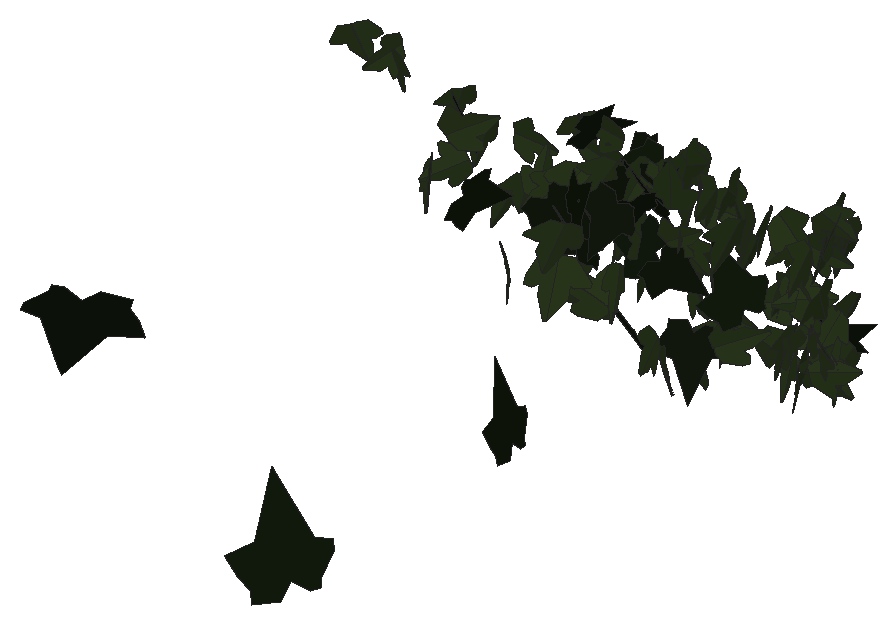
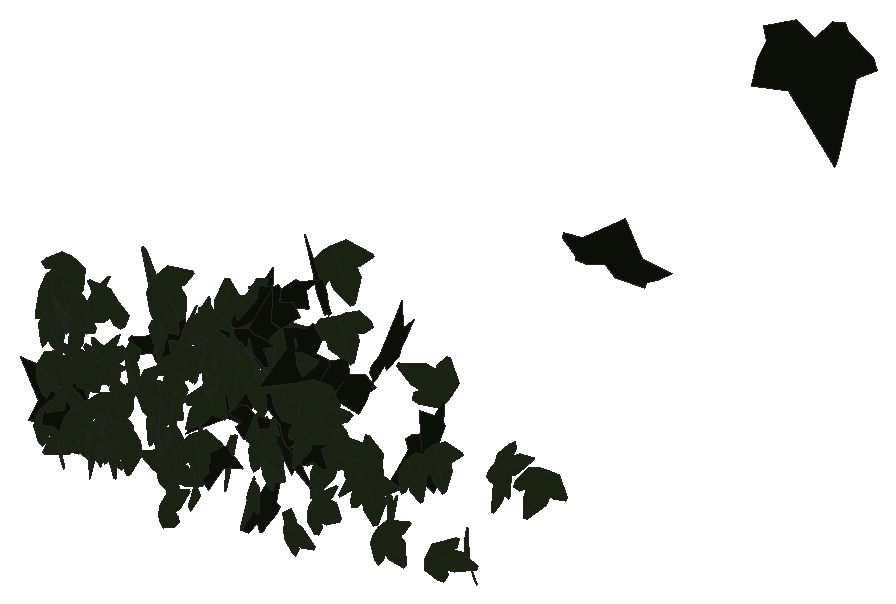
# SketchUp Ruby script. Lengths in inches.
U = 1.inch
M = Sketchup.active_model
def pt(a) = Geom::Point3d.new(a.map { |v| v * U })
def face(e, loops, mat)
  f = e.add_face(loops[0].map { |a| pt(a) })
  loops[1..].each { |l| e.add_face(l.map { |a| pt(a) }).erase! }
  f.material = f.back_material = mat if mat
  f
end
# faces: each face lists its corners as indices into pts; further lists are holes
def faces(e, pts, list, mat = nil) = list.each { |f| face(e, (f[0].is_a?(Array) ? f : [f]).map { |l| l.map { |i| pts[i] } }, mat) }
# xy, xz, yz: faces in a plane at the given z, y or x. An outline is a flat list of corners, or four numbers for a rectangle; further outlines are holes
def ring(l) = l.size == 4 ? [[l[0], l[1]], [l[2], l[1]], [l[2], l[3]], [l[0], l[3]]] : l.each_slice(2).to_a
def flat(e, list, mat, &to3) = list.each { |f| face(e, (f[0].is_a?(Array) ? f : [f]).map { |l| ring(l).map { |u, v| to3.(u, v) } }, mat) }
def xy(e, z, list, mat = nil) = flat(e, list, mat) { |x, y| [x, y, z] }
def xz(e, y, list, mat = nil) = flat(e, list, mat) { |x, z| [x, y, z] }
def yz(e, x, list, mat = nil) = flat(e, list, mat) { |y, z| [x, y, z] }
def lines(e, pts, list) = list.each { |a, b| e.add_line(pt(pts[a]), pt(pts[b])) }
# prism: a flat outline (further loops are holes) pulled along v
def prism(e, loops, v, mat = nil)
  f = face(e, loops, mat); d = Geom::Vector3d.new(v.map { |x| x * U })
  f.pushpull(f.normal.samedirection?(d) ? d.length : -d.length)
end
def box(e, o, s, mat = nil) = prism(e, [[o, [o[0] + s[0], o[1], o[2]], [o[0] + s[0], o[1] + s[1], o[2]], [o[0], o[1] + s[1], o[2]]]], [0, 0, s[2]], mat)
def at(x, y, z, deg = 0) = Geom::Transformation.translation(pt([x, y, z])) * Geom::Transformation.rotation(ORIGIN, Z_AXIS, deg.degrees)
def axes(o, x, y, z) = Geom::Transformation.new([*x, 0, *y, 0, *z, 0, *pt(o).to_a, 1])
def part(name) = M.definitions.add(name)
# library, detail: a bought-in or finely detailed component or shape, given as its bounding box
def library(name, o, s) = part(name).tap { |d| box(d.entities, o, s) }
def detail(e, o, s) = box(e.add_group.entities, o, s)
def put(e, d, t, mat = nil) = e.add_instance(d, t).tap { |i| i.material = mat if mat }
def group(e, t, mat = nil) = e.add_group.tap { |g| g.transformation = t; g.material = mat if mat }.entities
root = M.entities
M.materials.add("efeu1").color = [18, 25, 13]
M.materials.add("efeu2").color = [43, 57, 29]
c1 = part("ivyleaf_9")
p = [[1.54,2.16,1.25],[1.36,2.04,1.19],[-0.21,0.99,0.68],[-0.71,1.11,0.82],[-0.85,0.86,0.67],[-0.8,0.17,0.21],
  [-0.9,-0.01,0.1],[-0.67,-0.16,-0.02],[-0.08,-0.08,-0.05],[-0.03,-0.6,-0.4],[0.65,-0.88,-0.66],[0.83,-0.6,-0.49],
  [1.29,-0.42,-0.43],[1.8125,-0.07,-0.26],[1.21,0.44,0.15]]
faces(c1.entities,p,[[0,1,2,3,4,5,6,7,8,9,10,11,12,13,14]],"efeu1")
c2 = part("ivyleaf_10")
p = [[0,0.5,-0.03],[-0.0625,2.02,-0.43],[-0.19,2.01,-0.46],[-0.54,1.05,-0.29],[-0.52,0.625,-0.18],[-0.83,0.76,-0.28],
  [-1.16,0.64,-0.33],[-1.15,0.33,-0.24],[-0.77,-0.39,0.02],[-0.3,-0.51,0.16],[0.04,-0.48,0.23],[-0.02,2.01,-0.4375],
  [-0.06,2.01,-0.43],[0.04,-0.49,0.23],[0.67,-0.49,0.14],[1.38,0.36,-0.2],[1.375,0.51,-0.24],[0.81,0.65,-0.19],
  [0.62,0.59,-0.15],[0.6,1.09,-0.28],[0.5,1.23,-0.31]]
faces(c2.entities,p,[[0,1,2,3,4,5,6,7,8,9,10],[11,12,0,13,14,15,16,17,18,19,20]],"efeu2")
put(root,c1,axes([502.76,113.14,166.2],[0.63244,0.88262,-0.81674],[-0.4951,-0.63807,-1.10132],[-1.17596,0.74332,0.02443]))
put(root,c1,axes([509.15,115.98,157.04],[-1.26753,-0.11528,0.14381],[0.14961,0.00424,1.22642],[-0.12419,1.18175,0.00963]))
put(root,c1,axes([509.9,126.54,157.74],[-0.12905,-0.74325,0.56709],[0.24711,0.50872,0.7733],[-0.96441,0.22981,0.12226]))
put(root,c2,axes([509.01,130.26,163.54],[-0.45484,-0.62688,0.27611],[-0.14286,-0.23089,-0.78521],[0.72124,-0.44107,0.0186]))
put(root,c2,axes([508.29,130.92,161.64],[0.6186,0.59597,-0.17145],[-0.12286,-0.11932,-0.85966],[-0.65642,0.58397,-0.00068]))
put(root,c1,axes([508,132.13,163.08],[-0.11361,0.32654,0.68893],[0.21953,-0.63048,0.35679],[0.76682,0.22888,-0.00007]))
put(root,c2,axes([509.58,132.42,161.15],[0.62014,-0.35844,0.2759],[0.23589,-0.15102,-0.70387],[0.41988,0.61423,-0.01205]))
put(root,c1,axes([509.11,132.97,163.34],[-0.33636,-0.60165,0.16807],[-0.08252,-0.14242,-0.70457],[0.66773,-0.32067,-0.00242]))
put(root,c2,axes([508.61,132.79,159.72],[0.32026,0.29936,0.67732],[-0.5943,-0.35655,0.43102],[0.49605,-0.62045,0.07911]))
put(root,c2,axes([510.35,133.33,158.47],[0.55725,-0.41938,-0.236],[-0.17229,0.16327,-0.69103],[0.48531,0.53951,0.02567]))
put(root,c1,axes([509.21,133.71,163.17],[0.13784,0.62288,-0.22727],[-0.05689,-0.21225,-0.66119],[-0.71063,0.13781,0.00884]))
put(root,c2,axes([510.51,133.74,157.55],[-0.47497,0.45089,0.29765],[-0.21835,0.20259,-0.65504],[-0.53385,-0.48402,0.0031]))
put(root,c1,axes([505.63,133.89,161.93],[-0.0439,-0.14962,-0.77155],[0.31276,0.68333,-0.15983],[0.75516,-0.29172,0.02134]))
put(root,c2,axes([512.77,134.55,163.07],[-0.10334,-0.73527,0.34378],[-0.04182,-0.34127,-0.74248],[0.81059,-0.11135,0.00552]))
put(root,c2,axes([509.08,134.52,164.03],[0.17112,0.44347,-0.44791],[-0.19418,-0.39233,-0.48893],[-0.63878,0.23806,0.02864]))
put(root,c2,axes([501.59,134.09,162.96],[-0.31468,-0.25699,0.66664],[0.50868,0.43092,0.40624],[-0.50169,0.59812,-0.00625]))
put(root,c1,axes([508.51,133.94,163.68],[0.03435,0.0646,-0.7024],[0.13751,0.66355,0.07224],[0.71973,-0.12986,0.01972]))
put(root,c2,axes([506.11,134.21,159.22],[-0.30045,-0.6959,-0.35345],[0.17015,0.31122,-0.7574],[0.76174,-0.344,0.02977]))
put(root,c1,axes([513.23,134.43,160.41],[-0.71941,-0.3952,0.04042],[0.05266,-0.012,0.82003],[-0.39375,0.72044,0.03582]))
put(root,c2,axes([513.62,134.3,163.61],[0.3742,-0.58447,-0.45342],[-0.24442,0.3819,-0.694],[0.69818,0.44695,0.00006]))
put(root,c1,axes([508.85,134.89,162.64],[0.67994,-0.40982,0.23307],[-0.20003,0.11962,0.79389],[-0.42692,-0.70875,-0.00077]))
put(root,c2,axes([512.63,134.27,158.8125],[-0.1722,-0.2198,0.69867],[0.42346,0.55573,0.27921],[-0.59761,0.45712,-0.00348]))
put(root,c2,axes([502.91,135.06,157.77],[-0.24543,0.14957,0.73666],[0.60331,-0.42307,0.2869],[0.4484,0.6511,0.0172]))
put(root,c1,axes([506.42,135.04,160.11],[0.1436,-0.69547,0.0659],[0.00129,0.06473,0.73626],[-0.75422,-0.13231,0.01381]))
put(root,c2,axes([507.27,135.05,163.17],[-0.34879,-0.56177,0.39572],[-0.20967,-0.33561,-0.66124],[0.65438,-0.40696,-0.00094]))
put(root,c1,axes([501.87,134.21,160.62],[-0.02601,0.15388,-0.76833],[-0.2657,0.72148,0.15349],[0.73717,0.26548,0.02821]))
put(root,c2,axes([509.69,135.1,162.81],[-0.69884,-0.42344,-0.02594],[-0.01628,-0.02319,0.81704],[-0.42392,0.69894,0.01139]))
put(root,c1,axes([510.56,135.21,158.05],[-0.50863,-0.46562,-0.37996],[0.28315,0.25339,-0.68956],[0.53009,-0.58212,0.00376]))
put(root,c2,axes([514.76,135.74,162.17],[-0.06277,-0.3232,0.67328],[0.34516,-0.61172,-0.26147],[0.66229,0.28818,0.20008]))
put(root,c1,axes([509.4375,135.03,160.43],[0.03261,-0.16919,-0.68484],[0.05456,0.65788,-0.17339],[0.73224,-0.04148,0.04341]))
put(root,c1,axes([507.77,135.82,156.68],[0.53818,-0.55853,0.0638],[-0.04252,0.04763,0.77562],[-0.56056,-0.53985,0.00242]))
put(root,c1,axes([500.41,135.98,162.21],[0.20601,-0.41465,0.62014],[0.23799,-0.57321,-0.46233],[0.70702,0.31377,-0.02507]))
put(root,c2,axes([515.69,135.34,161.25],[-0.00186,-0.64236,-0.35691],[-0.00636,0.35691,-0.64233],[0.73482,0.00146,-0.00646]))
put(root,c2,axes([509.45,135.51,161.05],[-0.35965,-0.1338,0.50197],[0.48203,0.18375,0.37323],[-0.24547,0.55686,-0.00254]))
put(root,c2,axes([510.64,135.65,156.45],[-0.43062,0.45422,0.11722],[0.07325,-0.09043,0.62851],[0.5001,0.40436,0.00887]))
put(root,c1,axes([508.54,136.04,163.38],[-0.69456,-0.30587,-0.09091],[0.08487,0.03286,-0.75892],[0.3076,-0.69971,0.0041]))
put(root,c2,axes([514.28,136.11,157.07],[0.08219,-0.45535,-0.49981],[0.14455,-0.48002,0.46109],[-0.6605,-0.16171,0.03871]))
put(root,c2,axes([510.46,136.25,162.76],[-0.09771,-0.0466,0.72839],[0.38966,-0.62473,0.0123],[0.61716,0.38705,0.10756]))
put(root,c1,axes([508.31,135.9,160.12],[-0.49256,-0.24603,-0.52245],[-0.44637,-0.27346,0.54961],[-0.36639,0.66392,0.03277]))
put(root,c2,axes([507.32,136.14,162.03],[-0.24988,-0.35753,0.52872],[-0.28449,-0.44589,-0.43597],[0.57135,-0.37838,0.01416]))
put(root,c2,axes([515.21,136.01,161.87],[0.15719,-0.64001,-0.20308],[0.06404,-0.19332,0.65885],[-0.66839,-0.16904,0.01537]))
put(root,c2,axes([507.68,136.17,160.2],[-0.24466,0.54231,0.45521],[0.18978,-0.41377,0.59493],[0.68213,0.30963,-0.00226]))
put(root,c1,axes([505.57,135.73,159.64],[-0.67893,-0.21061,0.3147],[0.30789,0.06907,0.71047],[-0.22045,0.74513,0.02309]))
put(root,c2,axes([514.97,136.1875,158.62],[-0.19972,-0.04855,0.73188],[0.6946,-0.25623,0.17255],[0.23567,0.71406,0.11168]))
put(root,c2,axes([509.44,136.36,161.77],[0.18407,-0.39832,0.53365],[0.31637,-0.43488,-0.43372],[0.58596,0.35992,0.06654]))
put(root,c2,axes([504.91,136.14,161.58],[0.55503,0.32084,-0.42443],[-0.38423,-0.18256,-0.64045],[-0.36803,0.67444,0.02855]))
put(root,c2,axes([508.58,135.55,162.85],[-0.08432,-0.20978,-0.66626],[0.22283,0.60653,-0.23271],[0.6931,-0.22052,-0.00624]))
put(root,c2,axes([508.26,135.76,162.48],[0.00385,0.00014,0.69704],[-0.65732,0.23193,0.00359],[-0.23192,-0.65733,0.00141]))
put(root,c2,axes([506.5,136.27,160.11],[-0.39587,-0.53806,-0.08489],[-0.03261,-0.08135,0.66764],[-0.54374,0.39661,0.02177]))
put(root,c2,axes([509.75,135.95,160.56],[-0.36927,-0.35019,-0.33316],[0.2699,0.20281,-0.50798],[0.43576,-0.42237,0.03231]))
put(root,c2,axes([514.43,136.54,160.15],[-0.03483,0.05289,0.64535],[-0.27547,-0.5861,0.03317],[0.586,-0.27237,0.05395]))
put(root,c2,axes([513.5625,136.46,158.56],[0.20561,-0.66087,0.29802],[0.10354,-0.27983,-0.69196],[0.71752,0.22975,0.01445]))
put(root,c2,axes([514.16,136.17,160.26],[0.20562,-0.11436,-0.72012],[0.72137,-0.07706,0.21822],[-0.10619,-0.74493,0.08798]))
put(root,c2,axes([515.6,136.26,159.97],[0.59977,-0.08531,-0.20905],[-0.20735,0.02668,-0.60581],[0.08935,0.6346,-0.00263]))
put(root,c2,axes([513.57,136.17,162.82],[0.46659,0.11586,0.59129],[0.57429,0.14078,-0.48076],[-0.18232,0.73994,-0.00112]))
put(root,c2,axes([504.04,136.3125,160.77],[0.51328,0.03697,-0.5499],[-0.54968,-0.0203,-0.51444],[-0.04007,0.75195,0.01315]))
put(root,c2,axes([513.59,136.38,157.62],[0.56688,-0.32942,0.126],[0.10541,-0.06937,-0.65561],[0.33657,0.57656,-0.00689]))
put(root,c2,axes([513.72,136.29,160.6],[0.29138,0.00595,0.60829],[0.60673,0.0458,-0.29108],[-0.04387,0.67292,0.01443]))
put(root,c2,axes([513.69,136.23,158.44],[-0.19042,-0.63364,-0.10714],[0.04502,0.09831,-0.66148],[0.64106,-0.19512,0.01463]))
put(root,c2,axes([515.59,135.93,162.73],[0.22256,-0.29941,0.51724],[-0.26569,0.44483,0.37182],[-0.53534,-0.34524,0.0305]))
put(root,c1,axes([507.7,136.25,163.02],[-0.68079,0.40892,0.16753],[-0.15229,0.07174,-0.79399],[-0.41484,-0.69742,0.01655]))
put(root,c2,axes([511.14,136.37,157.64],[-0.02455,-0.00322,0.68376],[-0.6544,-0.19826,-0.02443],[0.19825,-0.65485,0.00403]))
put(root,c2,axes([509.47,136.54,158.8],[0.11131,-0.06283,0.68473],[0.65079,-0.2143,-0.12546],[0.22198,0.65978,0.02446]))
put(root,c2,axes([511.58,136.43,159.35],[0.13411,-0.72065,0.02541],[0.00289,-0.02531,-0.73302],[0.72109,0.13412,-0.00179]))
put(root,c2,axes([514.98,136.27,157.79],[0.12019,-0.0061,-0.71282],[0.71223,0.03094,0.11983],[0.0295,-0.72222,0.01115]))
put(root,c2,axes([512.75,136.36,158.04],[-0.33329,0.06564,-0.65922],[0.65408,-0.08457,-0.33911],[-0.10519,-0.73383,-0.01989]))
put(root,c1,axes([505.5,135.79,163.63],[0.35688,0.4478,0.5238],[0.33325,0.40416,-0.57258],[-0.60319,0.48824,-0.00643]))
put(root,c2,axes([511.2,136.7,162.79],[-0.22234,0.17606,-0.62368],[0.391,-0.48939,-0.27754],[-0.51681,-0.446,0.05834]))
put(root,c2,axes([514.78,136.39,162.17],[0.01057,-0.04651,0.69636],[0.67818,0.16514,0.00074],[-0.16481,0.67658,0.04769]))
put(root,c2,axes([515.31,136.28,163.66],[-0.44934,-0.1857,-0.41301],[0.37651,0.17006,-0.48609],[0.2516,-0.58614,-0.01018]))
put(root,c2,axes([509.75,136.01,163.8],[0.08521,-0.31214,-0.62246],[0.0305,0.62817,-0.31084],[0.69567,0.0107,0.08987]))
put(root,c2,axes([506.2,136.5,163.4],[-0.16344,0.09841,-0.64148],[-0.64335,0.06241,0.17349],[0.08533,0.65902,0.07936]))
put(root,c2,axes([511.32,136.15,163.31],[0.03194,-0.47522,-0.52635],[-0.01219,0.52644,-0.47603],[0.70903,0.03046,0.01553]))
put(root,c2,axes([514.81,136.35,157.88],[-0.55346,-0.08744,-0.51833],[0.51138,0.08463,-0.56031],[0.12166,-0.75353,-0.00279]))
put(root,c2,axes([506.04,136.38,157.22],[0.00212,0.06646,0.66374],[-0.66611,0.03558,-0.00144],[-0.03555,-0.66279,0.06648]))
put(root,c2,axes([510.59,136.86,157.19],[0.06859,-0.15343,0.55243],[0.36363,-0.41337,-0.16605],[0.47364,0.33958,0.04748]))
put(root,c1,axes([505.58,136.66,161.64],[0.33775,-0.11441,-0.67583],[0.67314,0.19748,0.30298],[0.12929,-0.72926,0.18807]))
put(root,c2,axes([508.91,136.37,162.45],[-0.38907,0.28249,-0.46068],[-0.40035,0.24393,0.47532],[0.40208,0.51623,0.0275]))
put(root,c2,axes([512.88,136.98,159.75],[0.00838,-0.05996,0.64957],[0.3723,-0.53299,-0.05401],[0.53566,0.37139,0.02737]))
put(root,c2,axes([506.82,136.77,160.23],[-0.13343,-0.6181,0.25042],[-0.02977,-0.24961,-0.63195],[0.66623,-0.13495,0.02191]))
put(root,c1,axes([506.07,136.69,160.61],[-0.6226,0.34576,-0.33148],[0.28567,-0.16831,-0.71212],[-0.38448,-0.68496,0.00766]))
put(root,c2,axes([496.7,137.02,163.05],[0.06487,0.12347,-0.66154],[-0.25581,-0.6102,-0.13897],[-0.62245,0.26364,-0.01184]))
put(root,c2,axes([509.23,136.375,163.65],[-0.28923,-0.57839,-0.34318],[0.17542,0.29575,-0.64631],[0.64926,-0.33757,0.02175]))
put(root,c2,axes([498.15,136.93,159.18],[0.38476,-0.31679,0.534],[0.423,-0.32614,-0.49826],[0.45452,0.57169,0.01166]))
put(root,c2,axes([500.66,136.79,161.51],[-0.06195,-0.61475,0.18438],[0.01894,-0.18691,-0.61681],[0.64152,-0.05385,0.03601]))
put(root,c2,axes([505.86,136.77,162.09],[-0.38912,-0.02553,-0.61373],[-0.60901,-0.07879,0.3894],[-0.08017,0.72241,0.02078]))
put(root,c2,axes([515.01,136.15,159.35],[-0.09835,-0.24476,-0.67812],[0.23379,0.63659,-0.26367],[0.68198,-0.25352,-0.00741]))
put(root,c2,axes([515.08,136.66,159.14],[0.59464,-0.21924,-0.29688],[-0.27622,0.10899,-0.63374],[0.24476,0.65563,0.00608]))
put(root,c2,axes([506.36,137.08,159.875],[0.20806,-0.47597,0.46003],[0.17433,-0.4258,-0.5194],[0.63858,0.27132,-0.00809]))
put(root,c2,axes([510.11,137,159.05],[-0.02815,0.0607,-0.71661],[0.51489,-0.499,-0.06249],[-0.5021,-0.5151,-0.0239]))
put(root,c2,axes([514.99,137.05,157.32],[-0.08279,0.07986,0.75173],[0.64319,-0.38991,0.11226],[0.39722,0.64801,-0.0251]))
put(root,c2,axes([511.49,137.07,160.9],[0.10492,-0.48968,0.41911],[0.14561,-0.39564,-0.49871],[0.62788,0.17358,0.04562]))
put(root,c2,axes([508,136.6,162.65],[-0.20175,-0.63444,-0.20102],[0.0439,0.19691,-0.66552],[0.66407,-0.20577,-0.01708]))
put(root,c2,axes([502.35,136.8125,160.25],[-0.3491,-0.54002,0.09315],[-0.03784,-0.08643,-0.64286],[0.54669,-0.35082,0.01499]))
put(root,c2,axes([499.53,136.89,162.42],[-0.22005,-0.58774,0.10559],[-0.04041,-0.09762,-0.62757],[0.59578,-0.2237,-0.00357]))
put(root,c2,axes([515.5,137.15,158.36],[-0.0983,-0.54603,0.41116],[-0.03306,-0.4111,-0.55386],[0.68272,-0.09852,0.03238]))
put(root,c1,axes([514.96,136.73,158.87],[0.61619,0.35231,-0.28515],[0.23795,0.15814,0.70957],[0.38577,-0.6603,0.0178]))
put(root,c2,axes([515.55,137.2,160.16],[0.14815,-0.54853,0.36991],[0.0689,-0.36422,-0.56768],[0.658,0.16164,-0.02384]))
put(root,c2,axes([510.09,136.54,162.14],[0.18679,0.14994,0.59241],[0.37308,0.45503,-0.23365],[-0.51526,0.38383,0.04558]))
put(root,c2,axes([515.1875,136.57,158.13],[0.08533,-0.0376,-0.63001],[-0.44379,0.44846,-0.08687],[0.44876,0.45064,0.03389]))
put(root,c2,axes([512.98,137.375,161.48],[-0.11142,-0.12033,0.64185],[0.10955,-0.64535,-0.10197],[0.64378,0.08899,0.12844]))
put(root,c2,axes([510.59,136.91,158],[-0.08959,-0.0206,0.6802],[0.67819,0.0539,0.09095],[-0.05614,0.68395,0.01332]))
put(root,c2,axes([512.9,136.5,159.49],[-0.0386,-0.02389,0.66397],[0.35868,0.5591,0.04096],[-0.55926,0.36022,-0.01955]))
put(root,c2,axes([503.0625,136.47,160.34],[0.12316,0.56395,-0.45611],[0.03036,0.45822,0.57476],[0.72468,-0.11504,0.05343]))
put(root,c2,axes([510.65,137.33,159.39],[0.28966,-0.2534,0.61949],[0.51463,-0.34727,-0.38268],[0.42794,0.58913,0.04089]))
put(root,c2,axes([513.91,136.9,158.03],[0.2201,-0.54576,-0.24506],[-0.03148,0.25019,-0.58547],[0.59743,0.21425,0.05943]))
put(root,c2,axes([515.34,137.11,162.91],[-0.1854,-0.6431,0.00823],[-0.00231,-0.0079,-0.66929],[0.64314,-0.18542,-0.00003]))
put(root,c2,axes([514.24,137.3125,158.53],[0.19938,0.06023,-0.72349],[-0.68573,-0.23076,-0.20819],[-0.23841,0.71411,-0.00625]))
put(root,c2,axes([504.47,136.99,163.13],[-0.47457,-0.39617,-0.18142],[0.13796,0.11783,-0.6182],[0.41332,-0.49421,-0.00196]))
put(root,c2,axes([504.92,136.88,161.61],[-0.15972,-0.5508,-0.34731],[0.0802,0.33824,-0.5733],[0.6462,-0.17812,-0.01469]))
put(root,c2,axes([495.03,137.02,163.17],[-0.55717,-0.35067,-0.20841],[0.17795,0.10852,-0.65833],[0.36707,-0.58489,0.00281]))
put(root,c2,axes([496.64,137.04,162.79],[-0.59553,0.31842,-0.00472],[0.00402,-0.0025,-0.67531],[-0.31843,-0.59554,0.00031]))
put(root,c2,axes([508.96,137.59,163.06],[-0.1178,-0.38739,0.5028],[0.16927,-0.51204,-0.35486],[0.61174,0.06708,0.195]))
put(root,c2,axes([509.21,137.24,159.65],[-0.17822,-0.62832,-0.00984],[0.00292,0.00939,-0.6531],[0.62839,-0.17825,0.00024]))
put(root,c2,axes([511.875,137.39,161.9],[0.28532,-0.59955,0.11204],[0.06374,-0.0937,-0.66376],[0.60658,0.29185,0.01705]))
put(root,c2,axes([501.16,137.53,159.13],[-0.10787,-0.57396,0.34459],[-0.05457,-0.34034,-0.58396],[0.66723,-0.12063,0.00795]))
put(root,c2,axes([510.29,137,160.625],[0.19573,-0.5012,-0.38955],[-0.01182,0.4047,-0.52664],[0.63468,0.16211,0.11033]))
put(root,c2,axes([515.19,137.4375,162.21],[0.01987,-0.63703,0.16866],[0.00971,-0.16843,-0.63732],[0.6589,0.02169,0.0043]))
put(root,c2,axes([514.72,137.61,163.3],[0.31347,-0.42078,0.45178],[0.27538,-0.35818,-0.52468],[0.55256,0.41722,0.00519]))
put(root,c2,axes([508.9,137.41,163.14],[-0.30485,0.44976,-0.37554],[0.19077,-0.32407,-0.54299],[-0.55401,-0.35908,0.01967]))
put(root,c2,axes([510.07,137.73,157.04],[-0.03245,0.09547,0.64466],[0.19101,-0.61572,0.1008],[0.62307,0.19373,0.00268]))
put(root,c2,axes([507.13,136.89,158.45],[0.12288,-0.37507,-0.55074],[-0.02804,0.55662,-0.38533],[0.66574,0.09268,0.08542]))
put(root,c2,axes([503.8,137.72,159.32],[-0.04168,-0.39071,0.54145],[0.09114,-0.54075,-0.38319],[0.66145,0.04989,0.08692]))
put(root,c2,axes([501.83,137.22,161.48],[0.03804,-0.025,0.6654],[0.63589,0.19907,-0.02887],[-0.19752,0.63606,0.03519]))
put(root,c2,axes([498.81,137.7,159.25],[-0.1935,-0.12279,0.63408],[-0.31512,-0.55985,-0.20458],[0.56377,-0.35507,0.10329]))
